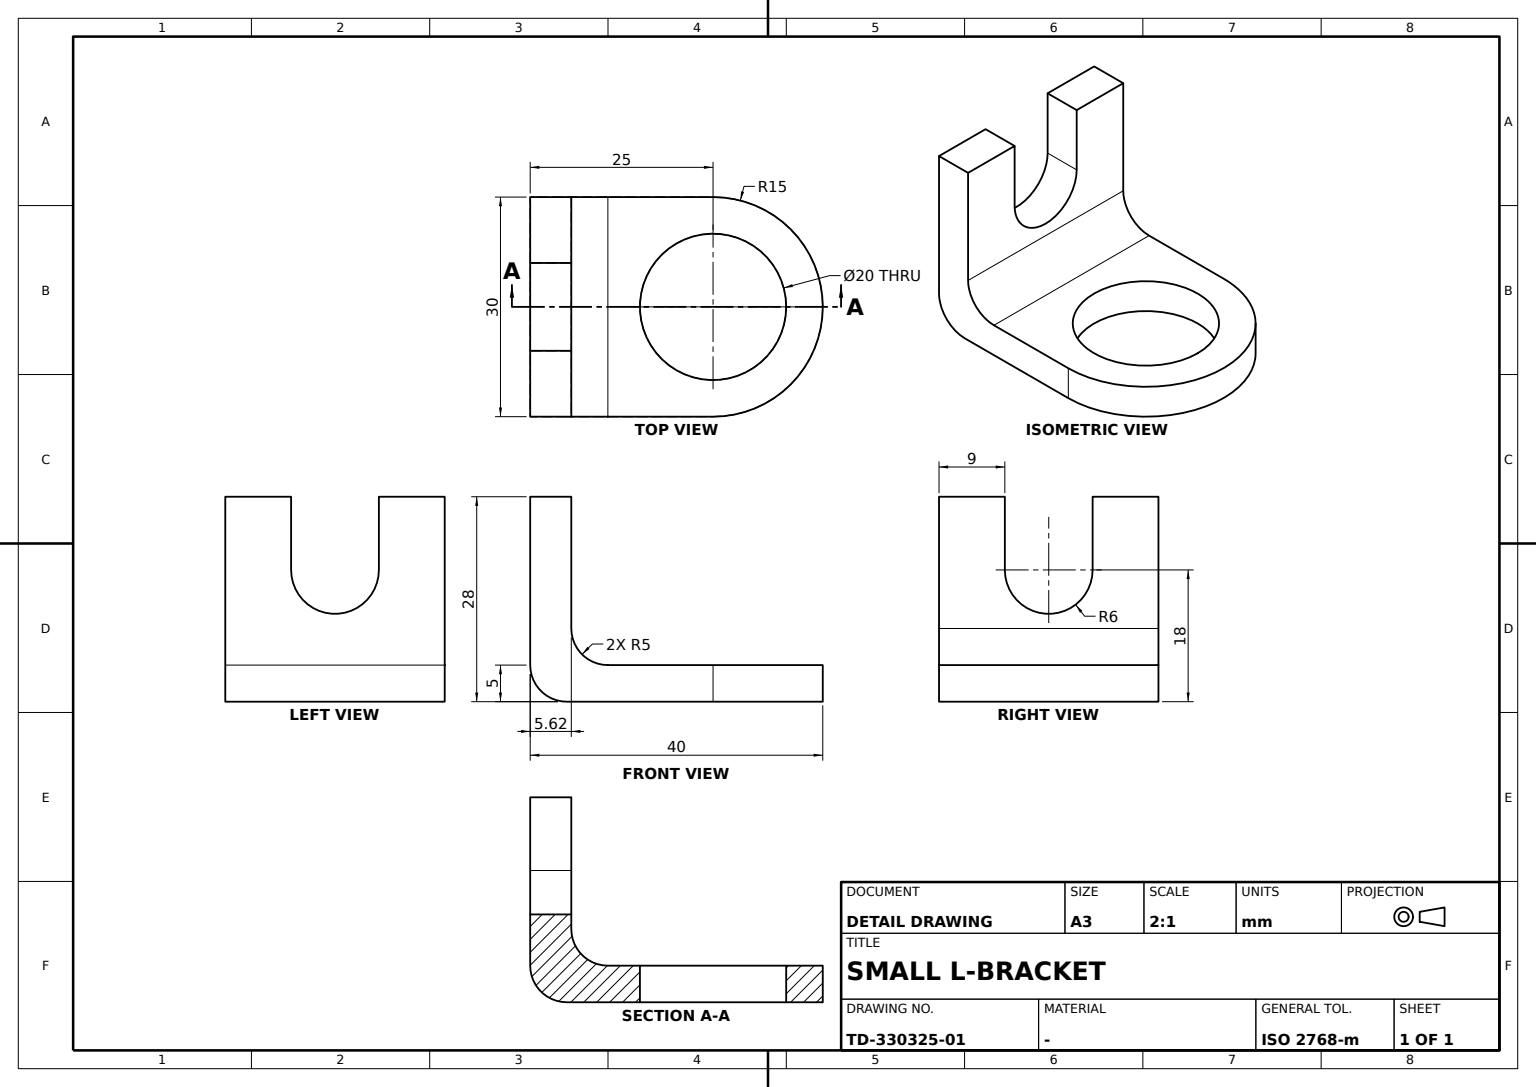
ISO-10303-21;
HEADER;
FILE_DESCRIPTION((''),'2;1');
FILE_NAME('','',(''),(''),'','','');
FILE_SCHEMA(('AUTOMOTIVE_DESIGN'));
ENDSEC;
DATA;
#1=APPLICATION_CONTEXT('');
#2=PRODUCT_CONTEXT('',#1,'mechanical');
#3=PRODUCT('','','',(#2));
#4=PRODUCT_DEFINITION_FORMATION('','',#3);
#5=PRODUCT_DEFINITION_CONTEXT('',#1,'design');
#6=PRODUCT_DEFINITION('','',#4,#5);
#7=PRODUCT_DEFINITION_SHAPE('','',#6);
#8=(LENGTH_UNIT()NAMED_UNIT(*)SI_UNIT(.MILLI.,.METRE.));
#9=(NAMED_UNIT(*)PLANE_ANGLE_UNIT()SI_UNIT($,.RADIAN.));
#10=(NAMED_UNIT(*)SI_UNIT($,.STERADIAN.)SOLID_ANGLE_UNIT());
#11=UNCERTAINTY_MEASURE_WITH_UNIT(LENGTH_MEASURE(0.005),#8,'distance_accuracy_value','');
#12=(GEOMETRIC_REPRESENTATION_CONTEXT(3)GLOBAL_UNCERTAINTY_ASSIGNED_CONTEXT((#11))GLOBAL_UNIT_ASSIGNED_CONTEXT((#8,#9,#10))REPRESENTATION_CONTEXT('',''));
#13=CARTESIAN_POINT('',(-25.,6.,28.));
#14=VERTEX_POINT('',#13);
#15=CARTESIAN_POINT('',(-25.,15.,28.));
#16=VERTEX_POINT('',#15);
#17=CARTESIAN_POINT('',(-25.,0.,28.));
#18=DIRECTION('',(0.,1.,0.));
#19=VECTOR('',#18,1000.);
#20=LINE('',#17,#19);
#21=EDGE_CURVE('',#14,#16,#20,.T.);
#22=ORIENTED_EDGE('',*,*,#21,.T.);
#23=CARTESIAN_POINT('',(-25.,15.,5.));
#24=VERTEX_POINT('',#23);
#25=CARTESIAN_POINT('',(-25.,15.,0.));
#26=DIRECTION('',(0.,0.,1.));
#27=VECTOR('',#26,1000.);
#28=LINE('',#25,#27);
#29=EDGE_CURVE('',#24,#16,#28,.T.);
#30=ORIENTED_EDGE('',*,*,#29,.F.);
#31=CARTESIAN_POINT('',(-25.,-15.,5.));
#32=VERTEX_POINT('',#31);
#33=CARTESIAN_POINT('',(-25.,0.,5.));
#34=LINE('',#33,#19);
#35=EDGE_CURVE('',#32,#24,#34,.T.);
#36=ORIENTED_EDGE('',*,*,#35,.F.);
#37=CARTESIAN_POINT('',(-25.,-15.,28.));
#38=VERTEX_POINT('',#37);
#39=CARTESIAN_POINT('',(-25.,-15.,0.));
#40=LINE('',#39,#27);
#41=EDGE_CURVE('',#32,#38,#40,.T.);
#42=ORIENTED_EDGE('',*,*,#41,.T.);
#43=CARTESIAN_POINT('',(-25.,-6.,28.));
#44=VERTEX_POINT('',#43);
#45=EDGE_CURVE('',#38,#44,#20,.T.);
#46=ORIENTED_EDGE('',*,*,#45,.T.);
#47=CARTESIAN_POINT('',(-25.,-6.,18.));
#48=VERTEX_POINT('',#47);
#49=CARTESIAN_POINT('',(-25.,-6.,0.));
#50=LINE('',#49,#27);
#51=EDGE_CURVE('',#48,#44,#50,.T.);
#52=ORIENTED_EDGE('',*,*,#51,.F.);
#53=CARTESIAN_POINT('',(-25.,6.,18.));
#54=VERTEX_POINT('',#53);
#55=CARTESIAN_POINT('',(-25.,0.,18.));
#56=DIRECTION('',(1.,0.,0.));
#57=DIRECTION('',(0.,0.,-1.));
#58=AXIS2_PLACEMENT_3D('',#55,#56,#57);
#59=CIRCLE('',#58,6.);
#60=EDGE_CURVE('',#54,#48,#59,.F.);
#61=ORIENTED_EDGE('',*,*,#60,.F.);
#62=CARTESIAN_POINT('',(-25.,6.,0.));
#63=LINE('',#62,#27);
#64=EDGE_CURVE('',#54,#14,#63,.T.);
#65=ORIENTED_EDGE('',*,*,#64,.T.);
#66=EDGE_LOOP('',(#22,#30,#36,#42,#46,#52,#61,#65));
#67=FACE_BOUND('',#66,.T.);
#68=AXIS2_PLACEMENT_3D('',#39,#56,#18);
#69=PLANE('',#68);
#70=ADVANCED_FACE('',(#67),#69,.F.);
#71=ORIENTED_EDGE('',*,*,#21,.F.);
#72=CARTESIAN_POINT('',(-19.380943,6.,28.));
#73=VERTEX_POINT('',#72);
#74=VECTOR('',#56,1000.);
#75=LINE('',#13,#74);
#76=EDGE_CURVE('',#14,#73,#75,.T.);
#77=ORIENTED_EDGE('',*,*,#76,.T.);
#78=CARTESIAN_POINT('',(-19.380943,15.,28.));
#79=VERTEX_POINT('',#78);
#80=CARTESIAN_POINT('',(-19.380943,0.,28.));
#81=DIRECTION('',(0.,-1.,0.));
#82=VECTOR('',#81,1000.);
#83=LINE('',#80,#82);
#84=EDGE_CURVE('',#79,#73,#83,.T.);
#85=ORIENTED_EDGE('',*,*,#84,.F.);
#86=CARTESIAN_POINT('',(0.,15.,28.));
#87=DIRECTION('',(-1.,0.,0.));
#88=VECTOR('',#87,1000.);
#89=LINE('',#86,#88);
#90=EDGE_CURVE('',#79,#16,#89,.T.);
#91=ORIENTED_EDGE('',*,*,#90,.T.);
#92=EDGE_LOOP('',(#71,#77,#85,#91));
#93=FACE_BOUND('',#92,.T.);
#94=CARTESIAN_POINT('',(0.,0.,28.));
#95=AXIS2_PLACEMENT_3D('',#94,#26,#18);
#96=PLANE('',#95);
#97=ADVANCED_FACE('',(#93),#96,.T.);
#98=CARTESIAN_POINT('',(-19.380943,6.,18.));
#99=VERTEX_POINT('',#98);
#100=CARTESIAN_POINT('',(-4.34,6.,18.));
#101=LINE('',#100,#88);
#102=EDGE_CURVE('',#54,#99,#101,.F.);
#103=ORIENTED_EDGE('',*,*,#102,.T.);
#104=LINE('',#98,#27);
#105=EDGE_CURVE('',#99,#73,#104,.T.);
#106=ORIENTED_EDGE('',*,*,#105,.T.);
#107=ORIENTED_EDGE('',*,*,#76,.F.);
#108=ORIENTED_EDGE('',*,*,#64,.F.);
#109=EDGE_LOOP('',(#103,#106,#107,#108));
#110=FACE_BOUND('',#109,.T.);
#111=AXIS2_PLACEMENT_3D('',#53,#18,#26);
#112=PLANE('',#111);
#113=ADVANCED_FACE('',(#110),#112,.F.);
#114=CARTESIAN_POINT('',(10.,0.,5.));
#115=VERTEX_POINT('',#114);
#116=CARTESIAN_POINT('',(0.,0.,5.));
#117=AXIS2_PLACEMENT_3D('',#116,#26,#56);
#118=CIRCLE('',#117,10.);
#119=EDGE_CURVE('',#115,#115,#118,.T.);
#120=ORIENTED_EDGE('',*,*,#119,.F.);
#121=EDGE_LOOP('',(#120));
#122=FACE_BOUND('',#121,.T.);
#123=CARTESIAN_POINT('',(-14.380943,15.,5.));
#124=VERTEX_POINT('',#123);
#125=CARTESIAN_POINT('',(-14.380943,-15.,5.));
#126=VERTEX_POINT('',#125);
#127=CARTESIAN_POINT('',(-14.380943,0.,5.));
#128=LINE('',#127,#82);
#129=EDGE_CURVE('',#124,#126,#128,.T.);
#130=ORIENTED_EDGE('',*,*,#129,.T.);
#131=CARTESIAN_POINT('',(0.,-15.,5.));
#132=VERTEX_POINT('',#131);
#133=LINE('',#131,#88);
#134=EDGE_CURVE('',#132,#126,#133,.T.);
#135=ORIENTED_EDGE('',*,*,#134,.F.);
#136=CARTESIAN_POINT('',(0.,15.,5.));
#137=VERTEX_POINT('',#136);
#138=CIRCLE('',#117,15.);
#139=EDGE_CURVE('',#132,#137,#138,.T.);
#140=ORIENTED_EDGE('',*,*,#139,.T.);
#141=LINE('',#136,#88);
#142=EDGE_CURVE('',#137,#124,#141,.T.);
#143=ORIENTED_EDGE('',*,*,#142,.T.);
#144=EDGE_LOOP('',(#130,#135,#140,#143));
#145=FACE_BOUND('',#144,.T.);
#146=AXIS2_PLACEMENT_3D('',#116,#26,#18);
#147=PLANE('',#146);
#148=ADVANCED_FACE('',(#122,#145),#147,.T.);
#149=CARTESIAN_POINT('',(0.,15.,0.));
#150=VERTEX_POINT('',#149);
#151=CARTESIAN_POINT('',(0.,15.,2.5));
#152=LINE('',#151,#27);
#153=EDGE_CURVE('',#150,#137,#152,.T.);
#154=ORIENTED_EDGE('',*,*,#153,.F.);
#155=CARTESIAN_POINT('',(-20.,15.,0.));
#156=VERTEX_POINT('',#155);
#157=LINE('',#149,#88);
#158=EDGE_CURVE('',#150,#156,#157,.T.);
#159=ORIENTED_EDGE('',*,*,#158,.T.);
#160=CARTESIAN_POINT('',(-20.,15.,5.));
#161=AXIS2_PLACEMENT_3D('',#160,#18,#26);
#162=CIRCLE('',#161,5.);
#163=EDGE_CURVE('',#156,#24,#162,.T.);
#164=ORIENTED_EDGE('',*,*,#163,.T.);
#165=ORIENTED_EDGE('',*,*,#29,.T.);
#166=ORIENTED_EDGE('',*,*,#90,.F.);
#167=CARTESIAN_POINT('',(-19.380943,15.,10.));
#168=VERTEX_POINT('',#167);
#169=CARTESIAN_POINT('',(-19.380943,15.,0.));
#170=LINE('',#169,#27);
#171=EDGE_CURVE('',#168,#79,#170,.T.);
#172=ORIENTED_EDGE('',*,*,#171,.F.);
#173=CARTESIAN_POINT('',(-14.380943,15.,10.));
#174=AXIS2_PLACEMENT_3D('',#173,#18,#26);
#175=CIRCLE('',#174,5.);
#176=EDGE_CURVE('',#124,#168,#175,.T.);
#177=ORIENTED_EDGE('',*,*,#176,.F.);
#178=ORIENTED_EDGE('',*,*,#142,.F.);
#179=EDGE_LOOP('',(#154,#159,#164,#165,#166,#172,#177,#178));
#180=FACE_BOUND('',#179,.T.);
#181=AXIS2_PLACEMENT_3D('',#149,#18,#87);
#182=PLANE('',#181);
#183=ADVANCED_FACE('',(#180),#182,.T.);
#184=CARTESIAN_POINT('',(-19.380943,-6.,28.));
#185=VERTEX_POINT('',#184);
#186=LINE('',#43,#74);
#187=EDGE_CURVE('',#44,#185,#186,.T.);
#188=ORIENTED_EDGE('',*,*,#187,.T.);
#189=CARTESIAN_POINT('',(-19.380943,-6.,18.));
#190=VERTEX_POINT('',#189);
#191=LINE('',#189,#27);
#192=EDGE_CURVE('',#190,#185,#191,.T.);
#193=ORIENTED_EDGE('',*,*,#192,.F.);
#194=CARTESIAN_POINT('',(-4.34,-6.,18.));
#195=LINE('',#194,#88);
#196=EDGE_CURVE('',#48,#190,#195,.F.);
#197=ORIENTED_EDGE('',*,*,#196,.F.);
#198=ORIENTED_EDGE('',*,*,#51,.T.);
#199=EDGE_LOOP('',(#188,#193,#197,#198));
#200=FACE_BOUND('',#199,.T.);
#201=AXIS2_PLACEMENT_3D('',#47,#18,#26);
#202=PLANE('',#201);
#203=ADVANCED_FACE('',(#200),#202,.T.);
#204=CARTESIAN_POINT('',(10.,0.,0.));
#205=VERTEX_POINT('',#204);
#206=CARTESIAN_POINT('',(0.,0.,0.));
#207=AXIS2_PLACEMENT_3D('',#206,#26,#56);
#208=CIRCLE('',#207,10.);
#209=EDGE_CURVE('',#205,#205,#208,.T.);
#210=ORIENTED_EDGE('',*,*,#209,.T.);
#211=EDGE_LOOP('',(#210));
#212=FACE_BOUND('',#211,.T.);
#213=ORIENTED_EDGE('',*,*,#158,.F.);
#214=CARTESIAN_POINT('',(0.,-15.,0.));
#215=VERTEX_POINT('',#214);
#216=CIRCLE('',#207,15.);
#217=EDGE_CURVE('',#215,#150,#216,.T.);
#218=ORIENTED_EDGE('',*,*,#217,.F.);
#219=CARTESIAN_POINT('',(-20.,-15.,0.));
#220=VERTEX_POINT('',#219);
#221=LINE('',#214,#88);
#222=EDGE_CURVE('',#215,#220,#221,.T.);
#223=ORIENTED_EDGE('',*,*,#222,.T.);
#224=CARTESIAN_POINT('',(-20.,0.,0.));
#225=LINE('',#224,#19);
#226=EDGE_CURVE('',#220,#156,#225,.T.);
#227=ORIENTED_EDGE('',*,*,#226,.T.);
#228=EDGE_LOOP('',(#213,#218,#223,#227));
#229=FACE_BOUND('',#228,.T.);
#230=AXIS2_PLACEMENT_3D('',#206,#26,#18);
#231=PLANE('',#230);
#232=ADVANCED_FACE('',(#212,#229),#231,.F.);
#233=ORIENTED_EDGE('',*,*,#176,.T.);
#234=CARTESIAN_POINT('',(-19.380943,-15.,10.));
#235=VERTEX_POINT('',#234);
#236=CARTESIAN_POINT('',(-19.380943,0.,10.));
#237=LINE('',#236,#82);
#238=EDGE_CURVE('',#168,#235,#237,.T.);
#239=ORIENTED_EDGE('',*,*,#238,.T.);
#240=CARTESIAN_POINT('',(-14.380943,-15.,10.));
#241=AXIS2_PLACEMENT_3D('',#240,#18,#26);
#242=CIRCLE('',#241,5.);
#243=EDGE_CURVE('',#126,#235,#242,.T.);
#244=ORIENTED_EDGE('',*,*,#243,.F.);
#245=ORIENTED_EDGE('',*,*,#129,.F.);
#246=EDGE_LOOP('',(#233,#239,#244,#245));
#247=FACE_BOUND('',#246,.T.);
#248=CARTESIAN_POINT('',(-14.380943,0.,10.));
#249=AXIS2_PLACEMENT_3D('',#248,#81,#57);
#250=CYLINDRICAL_SURFACE('',#249,5.);
#251=ADVANCED_FACE('',(#247),#250,.F.);
#252=ORIENTED_EDGE('',*,*,#192,.T.);
#253=CARTESIAN_POINT('',(-19.380943,-15.,28.));
#254=VERTEX_POINT('',#253);
#255=EDGE_CURVE('',#185,#254,#83,.T.);
#256=ORIENTED_EDGE('',*,*,#255,.T.);
#257=CARTESIAN_POINT('',(-19.380943,-15.,0.));
#258=LINE('',#257,#27);
#259=EDGE_CURVE('',#235,#254,#258,.T.);
#260=ORIENTED_EDGE('',*,*,#259,.F.);
#261=ORIENTED_EDGE('',*,*,#238,.F.);
#262=ORIENTED_EDGE('',*,*,#171,.T.);
#263=ORIENTED_EDGE('',*,*,#84,.T.);
#264=ORIENTED_EDGE('',*,*,#105,.F.);
#265=CARTESIAN_POINT('',(-19.380943,0.,18.));
#266=AXIS2_PLACEMENT_3D('',#265,#87,#26);
#267=CIRCLE('',#266,6.);
#268=EDGE_CURVE('',#99,#190,#267,.T.);
#269=ORIENTED_EDGE('',*,*,#268,.T.);
#270=EDGE_LOOP('',(#252,#256,#260,#261,#262,#263,#264,#269));
#271=FACE_BOUND('',#270,.T.);
#272=CARTESIAN_POINT('',(-19.380943,15.,5.));
#273=AXIS2_PLACEMENT_3D('',#272,#87,#81);
#274=PLANE('',#273);
#275=ADVANCED_FACE('',(#271),#274,.F.);
#276=ORIENTED_EDGE('',*,*,#119,.T.);
#277=EDGE_LOOP('',(#276));
#278=FACE_BOUND('',#277,.T.);
#279=ORIENTED_EDGE('',*,*,#209,.F.);
#280=EDGE_LOOP('',(#279));
#281=FACE_BOUND('',#280,.T.);
#282=CARTESIAN_POINT('',(0.,0.,4.9));
#283=AXIS2_PLACEMENT_3D('',#282,#57,#56);
#284=CYLINDRICAL_SURFACE('',#283,10.);
#285=ADVANCED_FACE('',(#278,#281),#284,.F.);
#286=ORIENTED_EDGE('',*,*,#163,.F.);
#287=ORIENTED_EDGE('',*,*,#226,.F.);
#288=CARTESIAN_POINT('',(-20.,-15.,5.));
#289=AXIS2_PLACEMENT_3D('',#288,#18,#26);
#290=CIRCLE('',#289,5.);
#291=EDGE_CURVE('',#220,#32,#290,.T.);
#292=ORIENTED_EDGE('',*,*,#291,.T.);
#293=ORIENTED_EDGE('',*,*,#35,.T.);
#294=EDGE_LOOP('',(#286,#287,#292,#293));
#295=FACE_BOUND('',#294,.T.);
#296=CARTESIAN_POINT('',(-20.,0.,5.));
#297=AXIS2_PLACEMENT_3D('',#296,#18,#57);
#298=CYLINDRICAL_SURFACE('',#297,5.);
#299=ADVANCED_FACE('',(#295),#298,.T.);
#300=ORIENTED_EDGE('',*,*,#268,.F.);
#301=ORIENTED_EDGE('',*,*,#102,.F.);
#302=ORIENTED_EDGE('',*,*,#60,.T.);
#303=ORIENTED_EDGE('',*,*,#196,.T.);
#304=EDGE_LOOP('',(#300,#301,#302,#303));
#305=FACE_BOUND('',#304,.T.);
#306=CARTESIAN_POINT('',(-4.34,0.,18.));
#307=AXIS2_PLACEMENT_3D('',#306,#87,#81);
#308=CYLINDRICAL_SURFACE('',#307,6.);
#309=ADVANCED_FACE('',(#305),#308,.F.);
#310=CARTESIAN_POINT('',(0.,-15.,2.5));
#311=LINE('',#310,#27);
#312=EDGE_CURVE('',#215,#132,#311,.T.);
#313=ORIENTED_EDGE('',*,*,#312,.T.);
#314=ORIENTED_EDGE('',*,*,#134,.T.);
#315=ORIENTED_EDGE('',*,*,#243,.T.);
#316=ORIENTED_EDGE('',*,*,#259,.T.);
#317=CARTESIAN_POINT('',(0.,-15.,28.));
#318=LINE('',#317,#74);
#319=EDGE_CURVE('',#38,#254,#318,.T.);
#320=ORIENTED_EDGE('',*,*,#319,.F.);
#321=ORIENTED_EDGE('',*,*,#41,.F.);
#322=ORIENTED_EDGE('',*,*,#291,.F.);
#323=ORIENTED_EDGE('',*,*,#222,.F.);
#324=EDGE_LOOP('',(#313,#314,#315,#316,#320,#321,#322,#323));
#325=FACE_BOUND('',#324,.T.);
#326=AXIS2_PLACEMENT_3D('',#214,#18,#87);
#327=PLANE('',#326);
#328=ADVANCED_FACE('',(#325),#327,.F.);
#329=ORIENTED_EDGE('',*,*,#45,.F.);
#330=ORIENTED_EDGE('',*,*,#319,.T.);
#331=ORIENTED_EDGE('',*,*,#255,.F.);
#332=ORIENTED_EDGE('',*,*,#187,.F.);
#333=EDGE_LOOP('',(#329,#330,#331,#332));
#334=FACE_BOUND('',#333,.T.);
#335=ADVANCED_FACE('',(#334),#96,.T.);
#336=ORIENTED_EDGE('',*,*,#153,.T.);
#337=ORIENTED_EDGE('',*,*,#139,.F.);
#338=ORIENTED_EDGE('',*,*,#312,.F.);
#339=ORIENTED_EDGE('',*,*,#217,.T.);
#340=EDGE_LOOP('',(#336,#337,#338,#339));
#341=FACE_BOUND('',#340,.T.);
#342=CARTESIAN_POINT('',(0.,0.,2.5));
#343=AXIS2_PLACEMENT_3D('',#342,#26,#18);
#344=CYLINDRICAL_SURFACE('',#343,15.);
#345=ADVANCED_FACE('',(#341),#344,.T.);
#346=CLOSED_SHELL('',(#70,#97,#113,#148,#183,#203,#232,#251,#275,#285,#299,#309,#328,#335,#345));
#347=MANIFOLD_SOLID_BREP('',#346);
#348=ADVANCED_BREP_SHAPE_REPRESENTATION('',(#347),#12);
#349=SHAPE_DEFINITION_REPRESENTATION(#7,#348);
ENDSEC;
END-ISO-10303-21;
